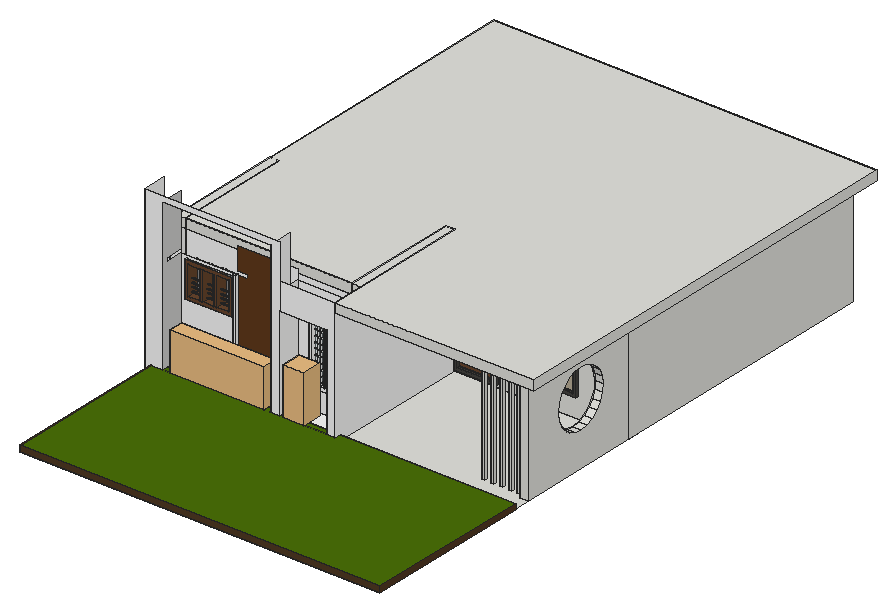
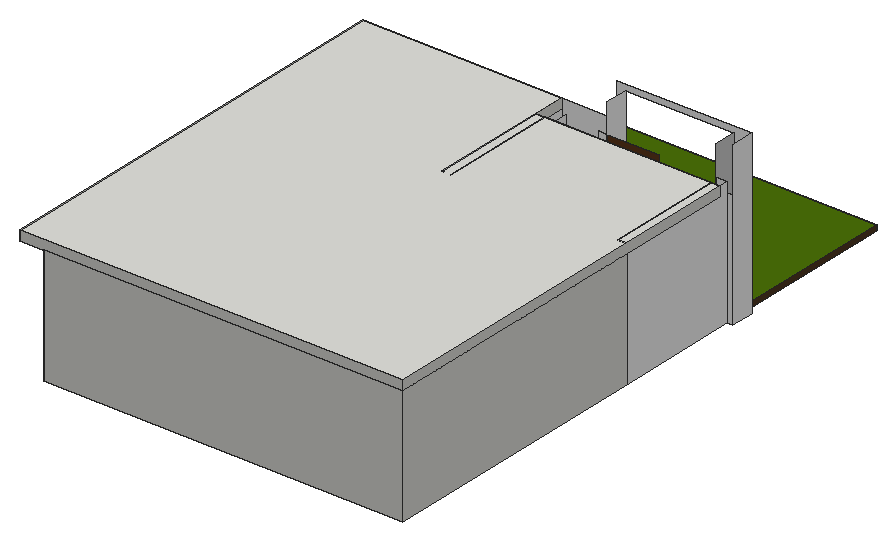
# SketchUp Ruby script. Lengths in inches.
U = 1.inch
M = Sketchup.active_model
def pt(a) = Geom::Point3d.new(a.map { |v| v * U })
def face(e, loops, mat)
  f = e.add_face(loops[0].map { |a| pt(a) })
  loops[1..].each { |l| e.add_face(l.map { |a| pt(a) }).erase! }
  f.material = f.back_material = mat if mat
  f
end
# faces: each face lists its corners as indices into pts; further lists are holes
def faces(e, pts, list, mat = nil) = list.each { |f| face(e, (f[0].is_a?(Array) ? f : [f]).map { |l| l.map { |i| pts[i] } }, mat) }
# xy, xz, yz: faces in a plane at the given z, y or x. An outline is a flat list of corners, or four numbers for a rectangle; further outlines are holes
def ring(l) = l.size == 4 ? [[l[0], l[1]], [l[2], l[1]], [l[2], l[3]], [l[0], l[3]]] : l.each_slice(2).to_a
def flat(e, list, mat, &to3) = list.each { |f| face(e, (f[0].is_a?(Array) ? f : [f]).map { |l| ring(l).map { |u, v| to3.(u, v) } }, mat) }
def xy(e, z, list, mat = nil) = flat(e, list, mat) { |x, y| [x, y, z] }
def xz(e, y, list, mat = nil) = flat(e, list, mat) { |x, z| [x, y, z] }
def yz(e, x, list, mat = nil) = flat(e, list, mat) { |y, z| [x, y, z] }
def lines(e, pts, list) = list.each { |a, b| e.add_line(pt(pts[a]), pt(pts[b])) }
# prism: a flat outline (further loops are holes) pulled along v
def prism(e, loops, v, mat = nil)
  f = face(e, loops, mat); d = Geom::Vector3d.new(v.map { |x| x * U })
  f.pushpull(f.normal.samedirection?(d) ? d.length : -d.length)
end
def box(e, o, s, mat = nil) = prism(e, [[o, [o[0] + s[0], o[1], o[2]], [o[0] + s[0], o[1] + s[1], o[2]], [o[0], o[1] + s[1], o[2]]]], [0, 0, s[2]], mat)
def at(x, y, z, deg = 0) = Geom::Transformation.translation(pt([x, y, z])) * Geom::Transformation.rotation(ORIGIN, Z_AXIS, deg.degrees)
def axes(o, x, y, z) = Geom::Transformation.new([*x, 0, *y, 0, *z, 0, *pt(o).to_a, 1])
def part(name) = M.definitions.add(name)
# library, detail: a bought-in or finely detailed component or shape, given as its bounding box
def library(name, o, s) = part(name).tap { |d| box(d.entities, o, s) }
def detail(e, o, s) = box(e.add_group.entities, o, s)
def put(e, d, t, mat = nil) = e.add_instance(d, t).tap { |i| i.material = mat if mat }
def group(e, t, mat = nil) = e.add_group.tap { |g| g.transformation = t; g.material = mat if mat }.entities
root = M.entities
M.materials.add("Brick_21_1K").color = [96, 58, 28]
M.materials.add("CALACATA").color = [248, 248, 247]
M.materials.add("GRANITO SIENA").color = [208, 208, 207]
M.materials.add("Glass_Mirror_01").color = [140, 140, 140]
M.materials.add("Glass_Mirror_1").color = [185, 173, 151]
M.materials.add("Glass_Safety_01").color = [204, 235, 244]
M.materials["Glass_Safety_01"].alpha = 0.25
M.materials.add("Metal_06_1K").color = [238, 236, 231]
M.materials.add("Wood_Planks_01_1K").color = [69, 67, 63]
M.materials.add("Wood_Veneer_15_1K").color = [103, 69, 45]
M.materials.add("[Groundcover_BarkChips]").color = [80, 57, 35]
M.materials.add("[Groundcover_RiverRock_4inch]").color = [80, 57, 35]
M.materials.add("[Groundcover_Rock_Crushed_2inch]").color = [74, 111, 8]
c1 = part("Untitled")
xy(c1.entities,0.3125,[[-290.45,43.1875,-283.67,49.67]],"[Groundcover_RiverRock_4inch]")
xy(c1.entities,0.6875,[[-290.45,43.1875,-283.67,49.67]],"[Groundcover_Rock_Crushed_2inch]")
xz(c1.entities,43.1875,[[-290.45,0.3125,-283.67,0.6875]],"[Groundcover_BarkChips]")
xz(c1.entities,49.67,[[-290.45,0.3125,-283.67,0.6875]],"[Groundcover_BarkChips]")
yz(c1.entities,-290.45,[[43.1875,0.3125,49.67,0.6875]],"[Groundcover_BarkChips]")
yz(c1.entities,-283.67,[[43.1875,0.3125,49.67,0.6875]],"[Groundcover_BarkChips]")
c2 = library("Group_2",[-1.28,-0.39,0],[21.22,20.51,48.44])
c3 = library("Planter with shrubs",[0,0,0],[56.02,15.3,25.28])
prism(root,[[[37.374,192.91,69.846],[37.374,193.576,69.846],[79.237,193.576,70.005],[79.237,192.91,70.005]]],[-0.002,0,0.464])
prism(root,[[[37.374,192.91,73.983],[37.374,193.576,73.983],[79.237,193.576,74.143],[79.237,192.91,74.143]]],[-0.002,0,0.464])
prism(root,[[[37.374,192.91,78.12],[37.374,193.576,78.12],[79.237,193.576,78.28],[79.237,192.91,78.28]]],[-0.002,0,0.464])
prism(root,[[[37.374,192.91,82.258],[37.374,193.576,82.258],[79.237,193.576,82.417],[79.237,192.91,82.417]]],[-0.002,0,0.464])
xy(root,0,[[16.353,3.987,385.657,131.734],[[16.353,131.734,384.753,131.734,384.753,320.734,205.353,320.734,205.353,191.734,16.353,191.734],[333.136,196.143,336.278,198.756],[342.231,196.143,345.373,198.756],[351.327,196.143,354.468,198.756],[360.422,196.143,363.563,198.756],[369.517,196.143,372.659,198.756]],[16.353,320.734,384.753,331.539]])
xy(root,0,[[10.353,167.734,148.353,191.734],[148.353,167.734,205.353,191.734],[25.353,200.734,196.353,320.734]],"CALACATA")
xy(root,6,[[28.353,167.734,139.353,167.734,139.353,191.734,86.143,191.734,86.143,189.734,83.143,189.734,83.143,191.734,28.353,191.734],[148.353,167.734,196.353,191.734],[83.143,189.734,86.143,191.734]],"CALACATA")
xy(root,28.368,[[161.803,188.734,180.978,191.734]],"CALACATA")
xy(root,31.368,[[164.803,188.734,177.978,188.734,177.978,192.234,175.185,192.234,175.185,191.734,174.685,191.734,174.685,192.234,171.891,192.234,171.891,191.734,171.391,191.734,171.391,192.234,168.597,192.234,168.597,191.734,168.097,191.734,168.097,192.234,164.803,192.234]],"CALACATA")
xy(root,33.864,[[164.803,191.734,168.097,192.234],[168.597,191.734,171.391,192.234],[171.891,191.734,174.685,192.234],[175.185,191.734,177.978,192.234]],"CALACATA")
xy(root,34.364,[[164.803,191.734,168.097,192.234],[168.597,191.734,171.391,192.234],[171.891,191.734,174.685,192.234],[175.185,191.734,177.978,192.234]],"CALACATA")
xy(root,39.707,[[164.803,191.734,168.097,192.234],[168.597,191.734,171.391,192.234],[171.891,191.734,174.685,192.234],[175.185,191.734,177.978,192.234]],"CALACATA")
xy(root,40.207,[[164.803,191.734,168.097,192.234],[168.597,191.734,171.391,192.234],[171.891,191.734,174.685,192.234],[175.185,191.734,177.978,192.234]],"CALACATA")
xy(root,45.549,[[164.803,191.734,168.097,192.234],[168.597,191.734,171.391,192.234],[171.891,191.734,174.685,192.234],[175.185,191.734,177.978,192.234]],"CALACATA")
xy(root,46.049,[[164.803,191.734,168.097,192.234],[168.597,191.734,171.391,192.234],[171.891,191.734,174.685,192.234],[175.185,191.734,177.978,192.234]],"CALACATA")
xy(root,51.392,[[164.803,191.734,168.097,192.234],[168.597,191.734,171.391,192.234],[171.891,191.734,174.685,192.234],[175.185,191.734,177.978,192.234]],"CALACATA")
xy(root,51.892,[[164.803,191.734,168.097,192.234],[168.597,191.734,171.391,192.234],[171.891,191.734,174.685,192.234],[175.185,191.734,177.978,192.234]],"CALACATA")
xy(root,57.234,[[164.803,191.734,168.097,192.234],[168.597,191.734,171.391,192.234],[171.891,191.734,174.685,192.234],[175.185,191.734,177.978,192.234]],"CALACATA")
xy(root,57.734,[[164.803,191.734,168.097,192.234],[168.597,191.734,171.391,192.234],[171.891,191.734,174.685,192.234],[175.185,191.734,177.978,192.234]],"CALACATA")
xy(root,63.077,[[164.803,191.734,168.097,192.234],[168.597,191.734,171.391,192.234],[171.891,191.734,174.685,192.234],[175.185,191.734,177.978,192.234]],"CALACATA")
xy(root,63.577,[[164.803,191.734,168.097,192.234],[168.597,191.734,171.391,192.234],[171.891,191.734,174.685,192.234],[175.185,191.734,177.978,192.234]],"CALACATA")
xy(root,68.919,[[164.803,191.734,168.097,192.234],[168.597,191.734,171.391,192.234],[171.891,191.734,174.685,192.234],[175.185,191.734,177.978,192.234]],"CALACATA")
xy(root,69.419,[[164.803,191.734,168.097,192.234],[168.597,191.734,171.391,192.234],[171.891,191.734,174.685,192.234],[175.185,191.734,177.978,192.234]],"CALACATA")
xy(root,74.762,[[164.803,191.734,168.097,192.234],[168.597,191.734,171.391,192.234],[171.891,191.734,174.685,192.234],[175.185,191.734,177.978,192.234]],"CALACATA")
xy(root,75.262,[[164.803,191.734,168.097,192.234],[168.597,191.734,171.391,192.234],[171.891,191.734,174.685,192.234],[175.185,191.734,177.978,192.234]],"CALACATA")
xy(root,80.604,[[164.803,191.734,168.097,192.234],[168.597,191.734,171.391,192.234],[171.891,191.734,174.685,192.234],[175.185,191.734,177.978,192.234]],"CALACATA")
xy(root,81.104,[[164.803,191.734,168.097,192.234],[168.597,191.734,171.391,192.234],[171.891,191.734,174.685,192.234],[175.185,191.734,177.978,192.234]],"CALACATA")
xz(root,167.734,[[10.353,0,148.353,0,148.353,6,28.353,6,28.353,160,139.353,160,139.353,6,148.353,6,148.353,166,10.353,166],[148.353,0,205.353,0,205.353,130,148.353,130,148.353,102,196.353,102,196.353,6,148.353,6]],"CALACATA")
xz(root,188.734,[[[161.803,28.368,180.978,97.45],[164.803,31.368,177.978,94.45]]],"CALACATA")
xz(root,188.734,[[[34.49,64.361,82.353,64.543,82.216,100.524,34.353,100.342],[37.478,67.372,37.364,97.353,49.818,97.401,52.818,97.412,63.773,97.454,63.773,97.359,63.887,67.485,63.887,67.473,66.887,67.485,66.773,97.359,66.773,97.466,79.227,97.513,79.227,97.353,79.341,67.532,66.887,67.485,63.887,67.473,52.932,67.431,51.432,67.426,49.932,67.42]],[49.932,67.42,51.432,67.426,52.932,67.431,52.818,97.353,52.818,97.412,49.818,97.401,49.818,97.342]],"Wood_Veneer_15_1K")
xz(root,189.734,[[83.143,6,86.143,102.578]],"CALACATA")
xz(root,191.734,[[86.143,6,139.353,6,139.353,130,86.143,130,86.143,106.305,96.364,106.305,96.364,102.578,86.143,102.578]],"Brick_21_1K")
xz(root,191.734,[[10.353,0,16.353,120],[16.353,0,148.353,0,148.353,130,139.353,130,139.353,6,28.353,6,28.353,130,16.353,130],[[28.353,6,83.143,102.578],[34.49,64.361,34.353,100.342,82.216,100.524,82.353,64.543]],[[148.353,6,196.353,120],[161.803,28.368,180.978,97.45]],[168.097,39.707,168.597,40.207],
  [171.391,51.392,171.891,51.892],[174.685,51.392,175.185,51.892],[171.391,63.077,171.891,63.577]],"CALACATA")
xz(root,191.734,[[168.097,31.368,168.597,33.864],[171.391,31.368,171.891,33.864],[174.685,31.368,175.185,33.864],[164.803,33.864,168.097,34.364],[168.097,33.864,168.597,34.364],
  [168.597,33.864,171.391,34.364],[171.391,33.864,171.891,34.364],[171.891,33.864,174.685,34.364],[174.685,33.864,175.185,34.364],[175.185,33.864,177.978,34.364],
  [168.097,34.364,168.597,39.707],[171.391,34.364,171.891,39.707],[174.685,34.364,175.185,39.707],[164.803,39.707,168.097,40.207],[168.597,39.707,171.391,40.207],
  [171.391,39.707,171.891,40.207],[171.891,39.707,174.685,40.207],[174.685,39.707,175.185,40.207],[175.185,39.707,177.978,40.207],[168.097,40.207,168.597,45.549],
  [171.391,40.207,171.891,45.549],[174.685,40.207,175.185,45.549],[164.803,45.549,168.097,46.049],[168.097,45.549,168.597,46.049],[168.597,45.549,171.391,46.049],
  [171.391,45.549,171.891,46.049],[171.891,45.549,174.685,46.049],[174.685,45.549,175.185,46.049],[175.185,45.549,177.978,46.049],[168.097,46.049,168.597,51.392],
  [171.391,46.049,171.891,51.392],[174.685,46.049,175.185,51.392],[164.803,51.392,168.097,51.892],[168.097,51.392,168.597,51.892],[168.597,51.392,171.391,51.892],
  [171.891,51.392,174.685,51.892],[175.185,51.392,177.978,51.892],[168.097,51.892,168.597,57.234],[171.391,51.892,171.891,57.234],[174.685,51.892,175.185,57.234],
  [164.803,57.234,168.097,57.734],[168.097,57.234,168.597,57.734],[168.597,57.234,171.391,57.734],[171.391,57.234,171.891,57.734],[171.891,57.234,174.685,57.734],
  [174.685,57.234,175.185,57.734],[175.185,57.234,177.978,57.734],[168.097,57.734,168.597,63.077],[171.391,57.734,171.891,63.077],[174.685,57.734,175.185,63.077],
  [164.803,63.077,168.097,63.577],[168.097,63.077,168.597,63.577],[168.597,63.077,171.391,63.577],[171.891,63.077,174.685,63.577],[174.685,63.077,175.185,63.577],
  [175.185,63.077,177.978,63.577],[168.097,63.577,168.597,68.919],[171.391,63.577,171.891,68.919],[174.685,63.577,175.185,68.919],[164.803,68.919,168.097,69.419],
  [168.097,68.919,168.597,69.419],[168.597,68.919,171.391,69.419],[171.391,68.919,171.891,69.419],[171.891,68.919,174.685,69.419],[174.685,68.919,175.185,69.419],
  [175.185,68.919,177.978,69.419],[168.097,69.419,168.597,74.762],[171.391,69.419,171.891,74.762],[174.685,69.419,175.185,74.762],[164.803,74.762,168.097,75.262],
  [168.097,74.762,168.597,75.262],[168.597,74.762,171.391,75.262],[171.391,74.762,171.891,75.262],[171.891,74.762,174.685,75.262],[174.685,74.762,175.185,75.262],
  [175.185,74.762,177.978,75.262],[168.097,75.262,168.597,80.604],[171.391,75.262,171.891,80.604],[174.685,75.262,175.185,80.604],[164.803,80.604,168.097,81.104],
  [168.097,80.604,168.597,81.104],[168.597,80.604,171.391,81.104],[171.391,80.604,171.891,81.104],[171.891,80.604,174.685,81.104],[174.685,80.604,175.185,81.104],
  [175.185,80.604,177.978,81.104],[168.097,81.104,168.597,86.447],[171.391,81.104,171.891,86.447],[174.685,81.104,175.185,86.447]],"Metal_06_1K")
xz(root,192.234,[[164.803,31.368,168.097,33.864],[168.597,31.368,171.391,33.864],[171.891,31.368,174.685,33.864],[175.185,31.368,177.978,33.864],[164.803,34.364,168.097,39.707],
  [168.597,34.364,171.391,39.707],[171.891,34.364,174.685,39.707],[175.185,34.364,177.978,39.707],[164.803,40.207,168.097,45.549],[168.597,40.207,171.391,45.549],
  [171.891,40.207,174.685,45.549],[175.185,40.207,177.978,45.549],[164.803,46.049,168.097,51.392],[168.597,46.049,171.391,51.392],[171.891,46.049,174.685,51.392],
  [175.185,46.049,177.978,51.392],[164.803,51.892,168.097,57.234],[168.597,51.892,171.391,57.234],[171.891,51.892,174.685,57.234],[175.185,51.892,177.978,57.234],
  [164.803,57.734,168.097,63.077],[168.597,57.734,171.391,63.077],[171.891,57.734,174.685,63.077],[175.185,57.734,177.978,63.077],[164.803,63.577,168.097,68.919],
  [168.597,63.577,171.391,68.919],[171.891,63.577,174.685,68.919],[175.185,63.577,177.978,68.919],[164.803,69.419,168.097,74.762],[168.597,69.419,171.391,74.762],
  [171.891,69.419,174.685,74.762],[175.185,69.419,177.978,74.762],[164.803,75.262,168.097,80.604],[168.597,75.262,171.391,80.604],[171.891,75.262,174.685,80.604],
  [175.185,75.262,177.978,80.604],[164.803,81.104,168.097,86.447],[168.597,81.104,171.391,86.447],[171.891,81.104,174.685,86.447],[175.185,81.104,177.978,86.447]],"Glass_Safety_01")
xz(root,196.143,[[333.136,0,336.278,101.967],[342.231,0,345.373,101.967],[351.327,0,354.468,101.967],[360.422,0,363.563,101.967],[369.517,0,372.659,101.967]])
xz(root,198.756,[[333.136,0,336.278,101.967],[342.231,0,345.373,101.967],[351.327,0,354.468,101.967],[360.422,0,363.563,101.967],[369.517,0,372.659,101.967]])
xz(root,200.734,[[[25.353,0,196.353,130],[66.887,67.485,79.341,67.532,79.227,97.353,79.227,97.513,66.773,97.466,66.773,97.359],[37.478,67.372,49.932,67.42,49.818,97.342,49.818,97.401,37.364,97.353],[52.932,67.431,63.887,67.473,63.887,67.485,63.773,97.359,63.773,97.454,52.818,97.412,52.818,97.353]]],"CALACATA")
xz(root,200.734,[[37.478,67.372,49.932,67.42,49.818,97.401,37.364,97.353],[66.888,67.484,79.341,67.532,79.226,97.513,66.773,97.466],[52.818,67.485,63.887,97.353]],"Glass_Mirror_01")
xz(root,320.734,[[16.353,0,25.353,130],[196.353,0,205.353,130]],"CALACATA")
yz(root,10.353,[[167.734,0,191.734,166]],"CALACATA")
yz(root,16.353,[[191.734,0,320.734,130]],"CALACATA")
yz(root,25.353,[[200.734,0,320.734,130]],"CALACATA")
yz(root,28.353,[[167.734,6,191.734,6,191.734,102.578,173.734,102.578,173.734,106.305,191.734,106.305,191.734,160,167.734,160]],"GRANITO SIENA")
yz(root,63.887,[[188.734,67.473,200.734,67.485]],"CALACATA")
yz(root,83.143,[[189.734,6,191.734,102.578]],"CALACATA")
yz(root,86.143,[[189.734,6,191.734,102.578]],"CALACATA")
yz(root,139.353,[[167.734,6,191.734,160]],"CALACATA")
yz(root,148.353,[[167.734,0,191.734,6],[167.734,6,191.734,6,191.734,120,173.734,120,173.734,102,167.734,102]],"CALACATA")
yz(root,161.803,[[188.734,28.368,191.734,97.45]],"CALACATA")
yz(root,164.803,[[188.734,31.368,192.234,31.368,192.234,33.864,191.734,33.864,191.734,34.364,192.234,34.364,192.234,39.707,191.734,39.707,191.734,40.207,192.234,40.207,192.234,45.549,191.734,45.549,191.734,46.049,192.234,46.049,192.234,51.392,191.734,51.392,191.734,51.892,192.234,51.892,192.234,57.234,191.734,57.234,191.734,57.734,192.234,57.734,192.234,63.077,191.734,63.077,191.734,63.577,192.234,63.577,192.234,68.919,191.734,68.919,191.734,69.419,192.234,69.419,192.234,74.762,191.734,74.762,191.734,75.262,192.234,75.262,192.234,80.604,191.734,80.604,191.734,81.104,192.234,81.104,192.234,86.447,191.734,86.447,191.734,86.947,192.234,86.947,192.234,92.289,191.734,92.289,191.734,92.789,192.234,92.789,192.234,93.95,191.734,93.95,191.734,94.45,188.734,94.45]],"CALACATA")
yz(root,168.097,[[191.734,31.368,192.234,33.864],[191.734,34.364,192.234,39.707],[191.734,40.207,192.234,45.549],[191.734,46.049,192.234,51.392],[191.734,51.892,192.234,57.234],
  [191.734,57.734,192.234,63.077],[191.734,63.577,192.234,68.919],[191.734,69.419,192.234,74.762],[191.734,75.262,192.234,80.604],[191.734,81.104,192.234,86.447]],"CALACATA")
yz(root,168.597,[[191.734,31.368,192.234,33.864],[191.734,34.364,192.234,39.707],[191.734,40.207,192.234,45.549],[191.734,46.049,192.234,51.392],[191.734,51.892,192.234,57.234],
  [191.734,57.734,192.234,63.077],[191.734,63.577,192.234,68.919],[191.734,69.419,192.234,74.762],[191.734,75.262,192.234,80.604],[191.734,81.104,192.234,86.447]],"CALACATA")
yz(root,171.391,[[191.734,31.368,192.234,33.864],[191.734,34.364,192.234,39.707],[191.734,40.207,192.234,45.549],[191.734,46.049,192.234,51.392],[191.734,51.892,192.234,57.234],
  [191.734,57.734,192.234,63.077],[191.734,63.577,192.234,68.919],[191.734,69.419,192.234,74.762],[191.734,75.262,192.234,80.604],[191.734,81.104,192.234,86.447]],"CALACATA")
yz(root,171.891,[[191.734,31.368,192.234,33.864],[191.734,34.364,192.234,39.707],[191.734,40.207,192.234,45.549],[191.734,46.049,192.234,51.392],[191.734,51.892,192.234,57.234],
  [191.734,57.734,192.234,63.077],[191.734,63.577,192.234,68.919],[191.734,69.419,192.234,74.762],[191.734,75.262,192.234,80.604],[191.734,81.104,192.234,86.447]],"CALACATA")
yz(root,174.685,[[191.734,31.368,192.234,33.864],[191.734,34.364,192.234,39.707],[191.734,40.207,192.234,45.549],[191.734,46.049,192.234,51.392],[191.734,51.892,192.234,57.234],
  [191.734,57.734,192.234,63.077],[191.734,63.577,192.234,68.919],[191.734,69.419,192.234,74.762],[191.734,75.262,192.234,80.604],[191.734,81.104,192.234,86.447]],"CALACATA")
yz(root,175.185,[[191.734,31.368,192.234,33.864],[191.734,34.364,192.234,39.707],[191.734,40.207,192.234,45.549],[191.734,46.049,192.234,51.392],[191.734,51.892,192.234,57.234],
  [191.734,57.734,192.234,63.077],[191.734,63.577,192.234,68.919],[191.734,69.419,192.234,74.762],[191.734,75.262,192.234,80.604],[191.734,81.104,192.234,86.447]],"CALACATA")
yz(root,177.978,[[188.734,31.368,188.734,94.45,191.734,94.45,191.734,93.95,192.234,93.95,192.234,92.789,191.734,92.789,191.734,92.289,192.234,92.289,192.234,86.947,191.734,86.947,191.734,86.447,192.234,86.447,192.234,81.104,191.734,81.104,191.734,80.604,192.234,80.604,192.234,75.262,191.734,75.262,191.734,74.762,192.234,74.762,192.234,69.419,191.734,69.419,191.734,68.919,192.234,68.919,192.234,63.577,191.734,63.577,191.734,63.077,192.234,63.077,192.234,57.734,191.734,57.734,191.734,57.234,192.234,57.234,192.234,51.892,191.734,51.892,191.734,51.392,192.234,51.392,192.234,46.049,191.734,46.049,191.734,45.549,192.234,45.549,192.234,40.207,191.734,40.207,191.734,39.707,192.234,39.707,192.234,34.364,191.734,34.364,191.734,33.864,192.234,33.864,192.234,31.368]],"CALACATA")
yz(root,180.978,[[188.734,28.368,191.734,97.45]],"CALACATA")
yz(root,196.353,[[200.734,0,320.734,130],[167.734,6,167.734,102,173.734,102,173.734,120,191.734,120,191.734,6]],"CALACATA")
yz(root,205.353,[[167.734,0,320.734,130]],"CALACATA")
yz(root,333.136,[[196.143,0,198.756,101.967]])
yz(root,336.278,[[196.143,0,198.756,101.967]])
yz(root,342.231,[[196.143,0,198.756,101.967]])
yz(root,345.373,[[196.143,0,198.756,101.967]])
yz(root,351.327,[[196.143,0,198.756,101.967]])
yz(root,354.468,[[196.143,0,198.756,101.967]])
yz(root,360.422,[[196.143,0,198.756,101.967]])
yz(root,363.563,[[196.143,0,198.756,101.967]])
yz(root,369.517,[[196.143,0,198.756,101.967]])
yz(root,372.659,[[196.143,0,198.756,101.967]])
p = [[34.353,191.734,100.342],[34.49,191.734,64.361],[34.49,188.734,64.361],[34.353,188.734,100.342],[82.353,191.734,64.543],[82.353,188.734,64.543],
  [82.216,191.734,100.524],[82.216,188.734,100.524],[37.478,200.734,67.372],[37.364,200.734,97.353],[37.364,188.734,97.353],[37.478,188.734,67.372],
  [49.932,200.734,67.42],[49.932,188.734,67.42],[49.818,200.734,97.342],[49.818,188.734,97.342],[52.932,191.734,67.431],[52.932,200.734,67.431],
  [52.818,200.734,97.353],[52.818,188.734,97.353],[52.932,188.734,67.431],[63.887,191.734,67.473],[63.887,200.734,67.473],[63.887,188.734,67.473],
  [63.773,188.734,97.359],[63.773,200.734,97.359],[63.887,200.734,67.485],[63.887,188.734,67.485],[65.387,191.734,67.479],[65.387,188.734,67.479],
  [66.887,191.734,67.485],[66.887,188.734,67.485],[66.887,200.734,67.485],[66.773,200.734,97.359],[66.773,188.734,97.359],[79.341,191.734,67.532],
  [79.341,200.734,67.532],[79.341,188.734,67.532],[79.227,188.734,97.353],[79.227,200.734,97.353],[338.753,309.063,64.414],[338.753,309.063,101.967],
  [205.353,320.734,0],[384.753,320.734,0],[79.341,191.734,67.372],[52.932,191.734,67.426]]
faces(root,p,[[0,1,2,3],[1,4,5,2],[14,12,13,15],[24,25,26,27],[28,21,23,29],[30,28,29,31],[38,39,36,35,37]],"CALACATA")
faces(root,p,[[4,6,7,5],[8,9,10,11],[12,8,11,13],[16,17,18,19,20],[21,22,17,16,20,23],[31,30,32,33,34],[35,36,32,30,31,37]],"Wood_Veneer_15_1K")
lines(root,p,[[40,41],[42,43],[35,44],[16,45]])
g1 = group(root,at(16.35,320.73,0))
xy(g1,0,[[9,9,180,277.76],[180,9,189,277.76],[189,9,359.4,277.76]])
xy(g1,7.05,[[194.875,-8.67,238.4,-5.67]])
xy(g1,10.05,[[197.875,-8.67,235.4,-5.48]],"Wood_Planks_01_1K")
xy(g1,27.03,[[274.4,-11.67,322.4,-8.67]])
xy(g1,30.03,[[277.4,-11.67,291.4,-8.67],[294.4,-11.67,305.4,-8.67],[308.4,-11.67,319.4,-8.67]],"Wood_Planks_01_1K")
xy(g1,109.23,[[277.4,-11.67,291.4,-8.67],[294.4,-11.67,305.4,-8.67],[308.4,-11.67,319.4,-8.67]],"Wood_Planks_01_1K")
xy(g1,109.63,[[197.875,-8.67,235.4,-5.48]])
xy(g1,112.23,[[274.4,-11.67,322.4,-8.67]])
xy(g1,112.63,[[194.875,-8.67,238.4,-5.67]])
xy(g1,120,[[[0,0,368.4,286.76],[9,9,359.4,277.76]]])
xz(g1,-11.67,[[[274.4,27.03,322.4,112.23],[277.4,30.03,291.4,109.23],[308.4,30.03,319.4,109.23],[294.4,30.03,305.4,109.23]]],"Wood_Planks_01_1K")
xz(g1,-8.67,[[[274.4,27.03,322.4,112.23],[277.4,30.03,291.4,109.23],[308.4,30.03,319.4,109.23],[294.4,30.03,305.4,109.23]]])
xz(g1,-8.67,[[277.4,30.03,291.4,109.23],[294.4,30.03,305.4,109.23],[308.4,30.03,319.4,109.23]],"Glass_Mirror_1")
xz(g1,-8.67,[[[194.875,7.05,238.4,112.63],[197.875,10.05,235.4,109.63]]],"Wood_Planks_01_1K")
xz(g1,-5.67,[[[194.875,7.05,238.4,112.63],[197.875,10.05,235.4,109.63]]])
xz(g1,-5.48,[[197.875,10.05,235.4,109.63]],"Wood_Veneer_15_1K")
xz(g1,0,[[0,0,9,120],[9,0,180,120],[180,0,189,120],[189,0,368.4,120]])
xz(g1,9,[[9,0,180,120],[180,0,189,120],[189,0,359.4,120]])
xz(g1,277.76,[[9,0,180,120],[180,0,189,120],[189,0,359.4,120]])
xz(g1,286.76,[[0,0,368.4,120]])
yz(g1,0,[[0,0,286.76,120]])
yz(g1,9,[[9,0,277.76,120]])
yz(g1,194.875,[[-8.67,7.05,-5.67,112.63]])
yz(g1,197.875,[[-8.67,10.05,-5.48,109.63]],"Wood_Planks_01_1K")
yz(g1,235.4,[[-8.67,10.05,-5.48,109.63]],"Wood_Planks_01_1K")
yz(g1,238.4,[[-8.67,7.05,-5.67,112.63]],"Wood_Planks_01_1K")
yz(g1,274.4,[[-11.67,27.03,-8.67,112.23]])
yz(g1,277.4,[[-11.67,30.03,-8.67,109.23]],"Wood_Planks_01_1K")
yz(g1,291.4,[[-11.67,30.03,-8.67,109.23]])
yz(g1,294.4,[[-11.67,30.03,-8.67,109.23]],"Wood_Planks_01_1K")
yz(g1,305.4,[[-11.67,30.03,-8.67,109.23]])
yz(g1,308.4,[[-11.67,30.03,-8.67,109.23]],"Wood_Planks_01_1K")
yz(g1,319.4,[[-11.67,30.03,-8.67,109.23]])
yz(g1,322.4,[[-11.67,27.03,-8.67,112.23]],"Wood_Planks_01_1K")
yz(g1,359.4,[[9,0,277.76,120]])
yz(g1,368.4,[[0,0,286.76,120]])
g2 = group(root,at(16.35,191.73,120))
xy(g2,-120,[[359.4,0,368.4,129]])
xy(g2,0,[[[189,-24,189,9,0,9,0,415.76,392.4,415.76,392.4,-24],[359.4,0,368.4,129]],[359.4,0,368.4,129]])
xy(g2,10,[[189,-24,392.4,-24,392.4,415.76,0,415.76,0,9,189,9]])
xz(g2,-24,[[189,0,392.4,10]])
xz(g2,0,[[359.4,-120,368.4,0]])
xz(g2,9,[[0,0,189,10]])
xz(g2,129,[[359.4,-120,368.4,0]])
xz(g2,415.76,[[0,0,392.4,10]])
yz(g2,0,[[9,0,415.76,10]])
yz(g2,189,[[-24,0,9,10]])
yz(g2,359.4,[[[0,-120,129,0],[67.59,-84.37,75.18,-83.24,82.22,-80.1875,88.22,-75.42,92.79,-69.25,95.6,-62.12,96.48,-54.5,95.35,-46.91,92.3,-39.875,87.53,-33.87,81.36,-29.3,74.23,-26.49,66.61,-25.61,59.02,-26.74,51.99,-29.79,45.98,-34.56,41.41,-40.73,38.6,-47.86,37.72,-55.48,38.85,-63.07,41.9,-70.1,46.68,-76.11,52.84,-80.68,59.97,-83.49]]])
yz(g2,368.4,[[[0,-120,129,0],[67.59,-84.37,59.97,-83.49,52.84,-80.68,46.68,-76.11,41.9,-70.1,38.85,-63.07,37.72,-55.48,38.6,-47.86,41.41,-40.73,45.98,-34.56,51.99,-29.79,59.02,-26.74,66.61,-25.61,74.23,-26.49,81.36,-29.3,87.53,-33.87,92.3,-39.875,95.35,-46.91,96.48,-54.5,95.6,-62.12,92.79,-69.25,88.22,-75.42,82.22,-80.1875,75.18,-83.24]]])
yz(g2,392.4,[[-24,0,415.76,10]])
p = [[368.4,59.97,-83.49],[368.4,67.59,-84.37],[359.4,67.59,-84.37],[359.4,59.97,-83.49],[368.4,75.18,-83.24],[359.4,75.18,-83.24],
  [368.4,52.84,-80.68],[359.4,52.84,-80.68],[368.4,82.22,-80.1875],[359.4,82.22,-80.1875],[368.4,46.68,-76.11],[359.4,46.68,-76.11],
  [368.4,88.22,-75.42],[359.4,88.22,-75.42],[368.4,41.9,-70.1],[359.4,41.9,-70.1],[368.4,92.79,-69.25],[359.4,92.79,-69.25],
  [368.4,38.85,-63.07],[359.4,38.85,-63.07],[368.4,95.6,-62.12],[359.4,95.6,-62.12],[368.4,37.72,-55.48],[359.4,37.72,-55.48],
  [368.4,96.48,-54.5],[359.4,96.48,-54.5],[368.4,38.6,-47.86],[359.4,38.6,-47.86],[368.4,95.35,-46.91],[359.4,95.35,-46.91],
  [368.4,41.41,-40.73],[359.4,41.41,-40.73],[368.4,92.3,-39.875],[359.4,92.3,-39.875],[368.4,45.98,-34.56],[359.4,45.98,-34.56],
  [368.4,87.53,-33.87],[359.4,87.53,-33.87],[368.4,51.99,-29.79],[359.4,51.99,-29.79],[368.4,81.36,-29.3],[359.4,81.36,-29.3],
  [368.4,59.02,-26.74],[359.4,59.02,-26.74],[368.4,74.23,-26.49],[359.4,74.23,-26.49],[368.4,66.61,-25.61],[359.4,66.61,-25.61]]
faces(g2,p,[[0,1,2,3],[1,4,5,2],[6,0,3,7],[4,8,9,5],[10,6,7,11],[8,12,13,9],[14,10,11,15],[12,16,17,13],
  [18,14,15,19],[16,20,21,17],[22,18,19,23],[20,24,25,21],[26,22,23,27],[24,28,29,25],[30,26,27,31],[28,32,33,29],
  [34,30,31,35],[32,36,37,33],[38,34,35,39],[36,40,41,37],[42,38,39,43],[40,44,45,41],[46,42,43,47],[44,46,47,45]])
put(root,c1,axes([15834.37,-1157.02,-4.49],[54.45967,0,0],[0,26.79148,0],[0,0,15.3576]))
put(root,c2,at(153.66,167.73,6))
put(root,c3,axes([35.48,167.73,6],[1.72862,0,0],[0,1,0],[0,0,1.547]))
